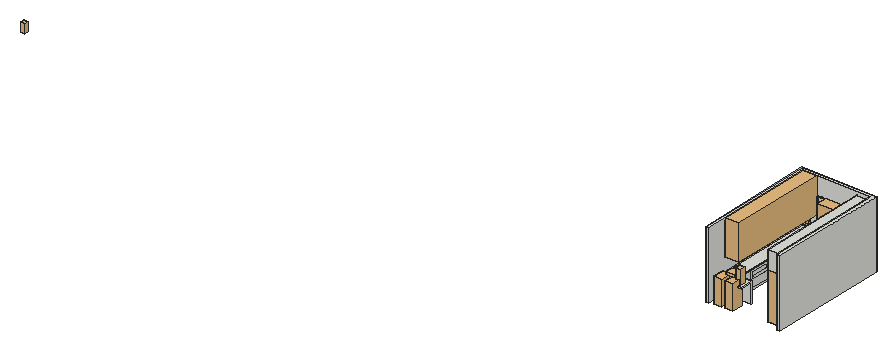
# SketchUp Ruby script. Lengths in inches.
U = 1.inch
M = Sketchup.active_model
def pt(a) = Geom::Point3d.new(a.map { |v| v * U })
def face(e, loops, mat)
  f = e.add_face(loops[0].map { |a| pt(a) })
  loops[1..].each { |l| e.add_face(l.map { |a| pt(a) }).erase! }
  f.material = f.back_material = mat if mat
  f
end
# faces: each face lists its corners as indices into pts; further lists are holes
def faces(e, pts, list, mat = nil) = list.each { |f| face(e, (f[0].is_a?(Array) ? f : [f]).map { |l| l.map { |i| pts[i] } }, mat) }
# xy, xz, yz: faces in a plane at the given z, y or x. An outline is a flat list of corners, or four numbers for a rectangle; further outlines are holes
def ring(l) = l.size == 4 ? [[l[0], l[1]], [l[2], l[1]], [l[2], l[3]], [l[0], l[3]]] : l.each_slice(2).to_a
def flat(e, list, mat, &to3) = list.each { |f| face(e, (f[0].is_a?(Array) ? f : [f]).map { |l| ring(l).map { |u, v| to3.(u, v) } }, mat) }
def xy(e, z, list, mat = nil) = flat(e, list, mat) { |x, y| [x, y, z] }
def xz(e, y, list, mat = nil) = flat(e, list, mat) { |x, z| [x, y, z] }
def yz(e, x, list, mat = nil) = flat(e, list, mat) { |y, z| [x, y, z] }
def lines(e, pts, list) = list.each { |a, b| e.add_line(pt(pts[a]), pt(pts[b])) }
# prism: a flat outline (further loops are holes) pulled along v
def prism(e, loops, v, mat = nil)
  f = face(e, loops, mat); d = Geom::Vector3d.new(v.map { |x| x * U })
  f.pushpull(f.normal.samedirection?(d) ? d.length : -d.length)
end
def box(e, o, s, mat = nil) = prism(e, [[o, [o[0] + s[0], o[1], o[2]], [o[0] + s[0], o[1] + s[1], o[2]], [o[0], o[1] + s[1], o[2]]]], [0, 0, s[2]], mat)
def at(x, y, z, deg = 0) = Geom::Transformation.translation(pt([x, y, z])) * Geom::Transformation.rotation(ORIGIN, Z_AXIS, deg.degrees)
def axes(o, x, y, z) = Geom::Transformation.new([*x, 0, *y, 0, *z, 0, *pt(o).to_a, 1])
def part(name) = M.definitions.add(name)
# library, detail: a bought-in or finely detailed component or shape, given as its bounding box
def library(name, o, s) = part(name).tap { |d| box(d.entities, o, s) }
def detail(e, o, s) = box(e.add_group.entities, o, s)
def put(e, d, t, mat = nil) = e.add_instance(d, t).tap { |i| i.material = mat if mat }
def group(e, t, mat = nil) = e.add_group.tap { |g| g.transformation = t; g.material = mat if mat }.entities
root = M.entities
M.materials.add("4 (5)").color = [147, 109, 57]
M.materials.add("[Translucent Glass Blue]").color = [100, 149, 237]
M.materials["[Translucent Glass Blue]"].alpha = 0.5
c1 = library("Dining chair\#1",[0,0,-0.11],[24.96,20.63,36.01])
c2 = library("Fridge",[0,0,0],[35.75,27.02,77.86])
c3 = part("Sink basin")
detail(c3.entities,[-0.15,-0.15,0],[19.98,14.07,5.91])
c4 = part("Untitled111")
put(c4.entities,c3,at(0.15,0.15,0),"4 (5)")
c5 = library("Blender",[2.53,2.84,0],[8.2,7.51,15.59])
c6 = library("mixer",[2.53,2.84,0],[8.2,7.51,15.59])
c7 = library("Cooker",[0,0,0],[12.41,9.47,7.59])
c8 = library("cooker1",[47.55,-42.3,30.26],[30,24.55,32.96])
c9 = library("5\#2",[-14.24,-10.22,0],[28.4,20.44,1.42])
c10 = library("chimney",[0,0,0],[35.95,27.65,32.08])
c11 = library("decoration wooden - glass bowl",[-0.13,0,1.29],[12.59,10.52,5.85])
c12 = library("Fruit bowl\#1",[0,0,0.08],[19.6875,19.6875,14.09])
c13 = library("Vase_Thin_Flowers",[-6.16,-5.72,0],[9.89,9.25,24.68])
c14 = part("Component\#4")
box(c14.entities,[0,0,0],[35.375,4.125,29.3125])
c15 = library("Knife Set",[-30.69,-30.94,0.125],[10.45,12.99,0.875])
c16 = library("5 STACKED BOWLS",[0,0,0],[6.24,6.24,7.68])
c17 = library("Jar",[0,0,0],[17.5625,21.24,23.15])
c18 = library("Kitchen utensils",[0,-7.04,-2.66],[17.4,17.6,7.97])
c19 = library("Microwave oven",[0,0,0],[23.78,13.12,19.55])
c20 = part("Group19\#1")
p = [[70.8125,1.1875,0],[1.1875,1.1875,0],[1.1875,46.8125,0],[70.8125,46.8125,0]]
lines(c20.entities,p,[[0,1],[1,2],[2,3],[3,0]])
c21 = part("Group18\#1")
prism(c21.entities,[[[72,48,0],[72,0,0],[0,0,0],[0,48,0]],[[1.1875,46.8125,0],[1.1875,1.1875,0],[70.8125,1.1875,0],[70.8125,46.8125,0]]],[0,0,5.875])
put(c21.entities,c20,at(0,0,0))
c22 = library("Group\#8",[30,0,0],[173,24.5,62.5])
xy(root,43.1875,[[54.6875,209,55.6875,214.875],[78.6875,209,78.6875,210.9375,79.1875,210.9375,79.1875,211.9375,78.6875,211.9375,78.6875,214.875,79.6875,214.875,79.6875,209],[31.1875,210.9375,54.6875,211.9375],[55.6875,210.9375,78.6875,211.9375],[78.6875,210.9375,79.1875,211.9375],
  [79.6875,210.9375,102.6875,211.9375],[102.6875,210.9375,103.1875,211.9375]])
xy(root,88.8125,[[54.6875,209,55.6875,214.875],[78.6875,209,79.6875,209,79.6875,214.875,78.6875,214.875,78.6875,211.9375,79.1875,211.9375,79.1875,210.9375,78.6875,210.9375],[31.1875,210.9375,54.6875,211.9375],[55.6875,210.9375,78.6875,211.9375],[78.6875,210.9375,79.1875,211.9375],
  [79.6875,210.9375,102.6875,211.9375],[102.6875,210.9375,103.1875,211.9375]])
xz(root,209,[[54.6875,43.1875,55.6875,88.8125],[78.6875,43.1875,79.6875,88.8125]])
xz(root,210.9375,[[31.1875,43.1875,54.6875,88.8125],[55.6875,43.1875,79.1875,88.8125],[79.6875,43.1875,103.1875,88.8125]])
xz(root,211.9375,[[31.1875,43.1875,54.6875,88.8125],[55.6875,43.1875,79.1875,88.8125],[79.6875,43.1875,103.1875,88.8125]])
xz(root,214.875,[[54.6875,43.1875,55.6875,88.8125],[78.6875,43.1875,79.6875,88.8125]])
yz(root,31.1875,[[210.9375,43.1875,211.9375,88.8125]])
yz(root,54.6875,[[209,43.1875,210.9375,88.8125],[210.9375,43.1875,214.875,88.8125]])
yz(root,55.6875,[[209,43.1875,210.9375,88.8125],[210.9375,43.1875,214.875,88.8125]])
yz(root,78.6875,[[209,43.1875,214.875,88.8125]])
yz(root,79.1875,[[210.9375,43.1875,211.9375,88.8125]])
yz(root,79.6875,[[209,43.1875,210.9375,88.8125],[210.9375,43.1875,214.875,88.8125]])
yz(root,103.1875,[[210.9375,43.1875,211.9375,88.8125]])
p = [[102,106,5],[102,106,82],[101.7,129,82],[101.7,129,5],[30,209,42],[30,209,90],
  [102,209,90],[102,209,42]]
faces(root,p,[[0,1,2,3]],"[Translucent Glass Blue]")
lines(root,p,[[4,5],[6,7],[7,4],[5,6]])
put(root,c1,axes([11.7,2.8125,0.02],[0,0.83304,0],[0.68983,0,0],[0,0,1.2069]))
put(root,c1,axes([31.83,2.8125,0.02],[0,0.83304,0],[0.68983,0,0],[0,0,1.2069]))
put(root,c2,axes([102,57.5,-0.78],[0,-1.28671,0],[0.88823,0,0],[0,0,1.06327]))
put(root,c4,at(100.48,80.02,7.05,-90))
put(root,c5,at(-1225.3125,-0.21,0))
put(root,c6,at(101.31,109.57,51))
put(root,c7,at(102,118.81,67))
put(root,c8,axes([123.29,116.6,0.26],[0,-0.74881,0],[0.50328,0,0],[0,0,0.60256]))
put(root,c9,at(61.42,194.74,34))
put(root,c10,at(46.62,189.4375,57.92))
put(root,c7,at(101.86,108.29,66.72))
put(root,c11,at(107.32,193.84,34))
put(root,c12,axes([20.35,19.08,35.44],[0.8,0,0],[0,0.8,0],[0,0,0.8]))
put(root,c13,axes([45.36,20.66,36],[1,0,0],[0,-1,0],[0,0,1]))
put(root,c14,axes([7.48,208.38,44.77],[0.33217,0,0],[0,0.15,0],[0,0,0.09327]))
put(root,c15,axes([38.45,208.6,70.17],[1,0,0],[0,0,1],[0,-1,0]))
put(root,c16,axes([105.875,113.05,34.99],[1.59,0,0],[0,1.59,0],[0,0,0.9222]))
put(root,c17,axes([110.72,121.59,19],[0.2556,0,0],[0,0.2556,0],[0,0,0.2556]))
put(root,c18,axes([7.16,78,38.95],[0,0,0.77],[0,-0.7182,0],[0.4356,0,0]))
put(root,c19,axes([113.48,58.5,39.05],[0,1,0],[-0.875,0,0],[0,0,1]))
put(root,c17,axes([110.72,113.72,19],[0.2556,0,0],[0,0.2556,0],[0,0,0.2556]))
g1 = group(root,at(6,36,0))
xy(g1,0,[[0,0,0,173,120,173,120,93.5,99,93.5,99,152,21,152,21,0]])
xy(g1,4,[[21,0,24,152],[96,93.5,99,149],[24,149,99,152]])
xy(g1,34,[[0,0,24,0,24,149,96,149,96,93.5,120,93.5,120,173,0,173]])
xz(g1,0,[[0,0,21,0,21,4,24,4,24,34,0,34],[24,33,24.13,33.02,24.25,33.07,24.35,33.15,24.43,33.25,24.48,33.37,24.5,33.5,24.48,33.63,24.43,33.75,24.35,33.85,24.25,33.93,24.13,33.98,24,34]])
xz(g1,93.5,[[99,0,120,0,120,34,96,34,96,4,99,4],[96,33,96,34,95.87,33.98,95.75,33.93,95.65,33.85,95.57,33.75,95.52,33.63,95.5,33.5,95.52,33.37,95.57,33.25,95.65,33.15,95.75,33.07,95.87,33.02]])
xz(g1,149,[[24,4,96,33],[24,33,24,34,24.13,33.98,24.25,33.93,24.35,33.85,24.43,33.75,24.48,33.63,24.5,33.5,24.48,33.37,24.43,33.25,24.35,33.15,24.25,33.07,24.13,33.02],[24,33,24.13,33.02,24.25,33.07,24.35,33.15,24.43,33.25,24.48,33.37,24.5,33.5,24.48,33.63,24.43,33.75,24.35,33.85,24.25,33.93,24.13,33.98,24,34,96,34,95.87,33.98,95.75,33.93,95.65,33.85,95.57,33.75,95.52,33.63,95.5,33.5,95.52,33.37,95.57,33.25,95.65,33.15,95.75,33.07,95.87,33.02,96,33],[96,33,95.87,33.02,95.75,33.07,95.65,33.15,95.57,33.25,95.52,33.37,95.5,33.5,95.52,33.63,95.57,33.75,95.65,33.85,95.75,33.93,95.87,33.98,96,34]])
xz(g1,152,[[21,0,99,4]])
xz(g1,173,[[0,0,120,34]])
yz(g1,0,[[0,0,173,34]])
yz(g1,21,[[0,0,152,4]])
yz(g1,24,[[0,4,149,33],[0,33,149,33,148.87,33.02,148.75,33.07,148.65,33.15,148.57,33.25,148.52,33.37,148.5,33.5,148.52,33.63,148.57,33.75,148.65,33.85,148.75,33.93,148.87,33.98,149,34,0,34],[149,33,149.13,33.02,149.25,33.07,149.35,33.15,149.43,33.25,149.48,33.37,149.5,33.5,149.48,33.63,149.43,33.75,149.35,33.85,149.25,33.93,149.13,33.98,149,34]])
yz(g1,96,[[93.5,4,149,33],[93.5,33,93.5,34,149,34,148.87,33.98,148.75,33.93,148.65,33.85,148.57,33.75,148.52,33.63,148.5,33.5,148.52,33.37,148.57,33.25,148.65,33.15,148.75,33.07,148.87,33.02,149,33]])
yz(g1,99,[[93.5,0,152,4]])
yz(g1,120,[[93.5,0,173,34]])
p = [[24.13,0,33.02],[24,0,33],[24,149,33],[24.13,149,33.02],[24.13,148.87,33.02],[24.25,0,33.07],
  [24.25,149,33.07],[24.25,148.75,33.07],[95.87,93.5,33.02],[95.75,93.5,33.07],[95.75,148.75,33.07],[95.75,149,33.07],
  [95.87,149,33.02],[95.87,148.87,33.02],[96,93.5,33],[96,149,33],[24,148.75,33.07],[24,148.87,33.02],
  [96,148.87,33.02],[96,148.75,33.07],[24.35,0,33.15],[24.35,149,33.15],[24.35,148.65,33.15],[24.43,0,33.25],
  [24.43,149,33.25],[24.43,148.57,33.25],[95.65,93.5,33.15],[95.57,93.5,33.25],[95.57,148.57,33.25],[95.57,149,33.25],
  [95.65,149,33.15],[95.65,148.65,33.15],[24,148.57,33.25],[24,148.65,33.15],[96,148.65,33.15],[96,148.57,33.25],
  [24.48,0,33.37],[24.48,149,33.37],[24.48,148.52,33.37],[95.52,93.5,33.37],[95.52,148.52,33.37],[95.52,149,33.37],
  [24,148.52,33.37],[96,148.52,33.37],[24.5,0,33.5],[24.5,149,33.5],[24.5,148.5,33.5],[95.5,93.5,33.5],
  [95.5,148.5,33.5],[95.5,149,33.5],[24,148.5,33.5],[96,148.5,33.5],[24.48,0,33.63],[24.48,149,33.63],
  [24.48,148.52,33.63],[95.52,93.5,33.63],[95.52,148.52,33.63],[95.52,149,33.63],[24,148.52,33.63],[96,148.52,33.63],
  [24.43,0,33.75],[24.43,149,33.75],[24.43,148.57,33.75],[95.57,93.5,33.75],[95.57,148.57,33.75],[95.57,149,33.75],
  [24,148.57,33.75],[96,148.57,33.75],[24.35,0,33.85],[24.35,149,33.85],[24.35,148.65,33.85],[95.65,93.5,33.85],
  [95.65,148.65,33.85],[95.65,149,33.85],[24,148.65,33.85],[96,148.65,33.85],[24.13,0,33.98],[24.25,0,33.93],
  [24.25,148.75,33.93],[24.25,149,33.93],[24.13,149,33.98],[24.13,148.87,33.98],[95.75,93.5,33.93],[95.75,148.75,33.93],
  [95.75,149,33.93],[95.87,93.5,33.98],[95.87,148.87,33.98],[95.87,149,33.98],[24,148.75,33.93],[96,148.75,33.93],
  [24,148.87,33.98],[96,148.87,33.98],[24,0,34],[24,149,34],[96,93.5,34],[96,149,34]]
faces(g1,p,[[0,1,2,3,4],[5,0,4,3,6,7],[8,9,10,11,12,13],[14,8,13,12,15],[16,17,4,13,18,19,10,7],[17,2,15,18,13,4],[20,5,7,6,21,22],[23,20,22,21,24,25],
  [26,27,28,29,30,31],[9,26,31,30,11,10],[32,33,22,31,34,35,28,25],[33,16,7,10,19,34,31,22],[36,23,25,24,37,38],[27,39,40,41,29,28],[42,32,25,28,35,43,40,38],[44,36,38,37,45,46],
  [39,47,48,49,41,40],[50,42,38,40,43,51,48,46],[52,44,46,45,53,54],[47,55,56,57,49,48],[58,50,46,48,51,59,56,54],[60,52,54,53,61,62],[55,63,64,65,57,56],[66,58,54,56,59,67,64,62],
  [68,60,62,61,69,70],[63,71,72,73,65,64],[74,66,62,64,67,75,72,70],[76,77,78,79,80,81],[77,68,70,69,79,78],[71,82,83,84,73,72],[82,85,86,87,84,83],[88,74,70,72,75,89,83,78],
  [90,88,78,83,89,91,86,81],[92,76,81,80,93],[85,94,95,87,86],[93,90,81,86,91,95]])
g2 = group(root,at(30,185.1,4))
xy(g2,0,[[0.5,-0.3,20.5,0],[21.5,-0.3,51.5,0],[52.5,-0.3,71,0],[0,-0.1,0.5,0],[20.5,-0.1,21.5,0],
  [51.5,-0.1,52.5,0],[71,-0.1,72,0]])
xy(g2,11.5,[[21.5,-0.3,51.5,-0.1]])
xy(g2,12.5,[[21.5,-0.3,51.5,-0.1]])
xy(g2,20.5,[[21.5,-0.3,51.5,-0.1],[52.5,-0.3,71,-0.1]])
xy(g2,21.5,[[21.5,-0.3,51.5,-0.1],[52.5,-0.3,71,-0.1]])
xy(g2,27.5,[[0.5,-0.3,11.5,-0.1],[11.5,-0.3,20.5,-0.1],[21.5,-0.3,51.5,-0.1],[52.5,-0.3,71,-0.1]])
xy(g2,29,[[0,-0.1,0.5,0],[0.5,-0.1,11.5,0],[11.5,-0.1,20.5,0],[20.5,-0.1,21.5,0],[21.5,-0.1,51.5,0],
  [51.5,-0.1,52.5,0],[52.5,-0.1,71,0],[71,-0.1,72,0]])
xz(g2,-0.3,[[0.5,0,20.5,27.5],[21.5,0,51.5,11.5],[52.5,0,71,20.5],[21.5,12.5,51.5,20.5],[21.5,21.5,51.5,27.5],
  [52.5,21.5,71,27.5]])
xz(g2,-0.1,[[[0,0,0.5,0,0.5,27.5,20.5,27.5,20.5,0,21.5,0,21.5,11.5,51.5,11.5,51.5,0,52.5,0,52.5,20.5,71,20.5,71,0,72,0,72,29,0,29],[21.5,12.5,51.5,20.5],[21.5,21.5,51.5,27.5],[52.5,21.5,71,27.5]]])
xz(g2,0,[[0,0,0.5,29]])
yz(g2,0,[[-0.1,0,0,29]])
yz(g2,0.5,[[-0.3,0,-0.1,27.5]])
yz(g2,20.5,[[-0.3,0,-0.1,27.5]])
yz(g2,21.5,[[-0.3,0,-0.1,11.5],[-0.3,12.5,-0.1,20.5],[-0.3,21.5,-0.1,27.5]])
yz(g2,51.5,[[-0.3,0,-0.1,11.5],[-0.3,12.5,-0.1,20.5],[-0.3,21.5,-0.1,27.5]])
yz(g2,52.5,[[-0.3,0,-0.1,20.5],[-0.3,21.5,-0.1,27.5]])
yz(g2,71,[[-0.3,0,-0.1,20.5],[-0.3,21.5,-0.1,27.5]])
yz(g2,72,[[-0.1,0,0,28.5],[-0.1,28.5,0,29]])
p = [[0.5,0,28.5],[0.5,-0.1,28.5],[0.5,0,27.5],[0.5,-0.1,27.5]]
lines(g2,p,[[0,1],[2,3]])
g3 = group(root,at(30,36,0))
xy(g3,0,[[0,24.5,0.1,66.5]])
xy(g3,4,[[0,0,0,24.5,0.1,24.5,0.1,23.5,0.3,23.5,0.3,0],[0.1,24.5,0.3,66.5],[0,66.5,0,87.5,0.1,87.5,0.1,87,0.3,87,0.3,67.5,0.1,67.5,0.1,66.5],[0,87.5,0,110,0.1,110,0.1,109.5,0.3,109.5,0.3,88.01,0.1,88.01,0.1,87.5],[0,110,0,130.5,0.1,130.5,0.1,130,0.3,130,0.3,110.5,0.1,110.5,0.1,110],
  [0,130.5,0,149,0.3,149,0.3,131,0.1,131,0.1,130.5]])
xy(g3,17,[[0.1,0,0.3,23.5],[0.1,24.5,0.3,66.5],[0.1,67.5,0.3,87],[0.1,88.01,0.3,109.5],[0.1,110.5,0.3,130],
  [0.1,131,0.3,149]])
xy(g3,18,[[0.1,0,0.3,23.5],[0.1,24.5,0.3,66.5],[0.1,110.5,0.3,130],[0.1,131,0.3,149]])
xy(g3,18.5,[[0.1,67.5,0.3,87],[0.1,88.01,0.3,109.5]])
xy(g3,22.3125,[[0.1,29.125,0.3,62.12]])
xy(g3,29.12,[[0.1,29.125,0.3,62.12]])
xy(g3,32,[[0.1,0,0.3,23.5],[0.1,67.5,0.3,87],[0.1,88,0.3,109.5],[0.1,110.5,0.3,130],[0.1,131,0.3,149]])
xy(g3,33,[[0,0,0.1,24.5],[0,24.5,0.3,66.5],[0,66.5,0.1,87.5],[0,87.5,0.1,110],[0,110,0.1,130.5],
  [0,130.5,0.1,149]])
xz(g3,0,[[0,4,0.3,4,0.3,17,0.1,17,0.1,17.5,0,17.5],[0,17.5,0.1,17.5,0.1,18,0.3,18,0.3,32,0,32],[0,32,0.1,33]])
xz(g3,23.5,[[0.1,4,0.3,17],[0.1,18,0.3,32]])
xz(g3,24.5,[[0,0,0.1,4],[0.1,4,0.3,17],[0.1,18,0.3,32],[0.1,32,0.3,33]])
xz(g3,29.125,[[0.1,22.3125,0.3,29.12]])
xz(g3,62.12,[[0.1,22.3125,0.3,29.12]])
xz(g3,66.5,[[0,0,0.1,4],[0.1,4,0.3,17],[0.1,18,0.3,18.5],[0.1,18.5,0.3,32],[0.1,32,0.3,33]])
xz(g3,67.5,[[0.1,4,0.3,17],[0.1,18.5,0.3,32]])
xz(g3,87,[[0.1,4,0.3,17],[0.1,18.5,0.3,32]])
xz(g3,88.01,[[0.1,4,0.3,17]])
xz(g3,109.5,[[0.1,4,0.3,17],[0.1,18.5,0.3,32]])
xz(g3,110.5,[[0.1,4,0.3,17],[0.1,18,0.3,32]])
xz(g3,130,[[0.1,4,0.3,17],[0.1,18,0.3,32]])
xz(g3,131,[[0.1,4,0.3,17],[0.1,18,0.3,32]])
xz(g3,149,[[0,4,0,32,0.3,32,0.3,18,0.1,18,0.1,17,0.3,17,0.3,4],[0,32,0.1,33]])
yz(g3,0,[[0,4,24.5,17.5]])
yz(g3,0.1,[[24.5,0,66.5,4],[[23.5,4,24.5,4,24.5,17,66.5,17,66.5,4,67.5,4,67.5,17,87,17,87,4,88.01,4,88.01,17,109.5,17,109.5,4,110.5,4,110.5,17,130,17,130,4,131,4,131,17,149,17,149,18,131,18,131,32,149,32,149,33,66.5,33,66.5,18,24.5,18,24.5,33,0,33,0,32,23.5,32,23.5,18,0,18,0,17,23.5,17],[88.01,18.5,88,32,109.5,32,109.5,18.5],[110.5,18,130,32],[67.5,18.5,87,32]],[29.125,22.3125,62.12,29.12]])
yz(g3,0.3,[[0,4,23.5,17],[24.5,4,66.5,17],[67.5,4,87,17],[88.01,4,109.5,17],[110.5,4,130,17],
  [131,4,149,17],[0,18,23.5,32],[[24.5,18,66.5,33],[29.125,22.3125,62.12,29.12]],[110.5,18,130,32],[131,18,149,32],
  [67.5,18.5,87,32],[88.01,18.5,109.5,18.5,109.5,32,88,32]])
p = [[0.1,88,32],[0.1,88.01,18.5],[0.3,88.01,18.5],[0.3,88,32]]
faces(g3,p,[[0,1,2,3]])
g4 = group(root,at(102.1,185,4))
xy(g4,0,[[-0.4,-55.5,0,-25.5],[-0.1,-25.5,-0.1,-24.5,-0.4,-24.5,-0.4,0,0,0,0,-25.5]])
xy(g4,13.5,[[-0.4,-55.5,-0.1,-25.5],[-0.1,-55.5,0,-25.5]])
xy(g4,14.5,[[-0.4,-55.5,-0.1,-25.5]])
xy(g4,28,[[-0.4,-55.5,-0.1,-25.5],[-0.1,-55.5,0,-25.5],[-0.4,-24.5,-0.1,0]])
xy(g4,29,[[-0.1,-55.5,0,-25.5],[-0.1,-25.5,0,0]])
xz(g4,-55.5,[[-0.4,0,0,13.5],[-0.1,13.5,0,14.5],[-0.4,14.5,0,28],[-0.1,28,0,29]])
xz(g4,-25.5,[[-0.4,0,-0.1,13.5],[-0.1,0,0,13.5],[-0.4,14.5,-0.1,28],[-0.1,14.5,0,28]])
xz(g4,-24.5,[[-0.4,0,-0.1,28]])
xz(g4,0,[[-0.4,0,0,28],[-0.1,28,0,29]])
yz(g4,-0.4,[[-55.5,0,-25.5,13.5],[-24.5,0,0,28],[-55.5,14.5,-25.5,28]])
yz(g4,-0.1,[[-25.5,0,-25.5,13.5,-55.5,13.5,-55.5,14.5,-25.5,14.5,-25.5,28,-55.5,28,-55.5,29,0,29,0,28,-24.5,28,-24.5,0]])
yz(g4,0,[[-55.5,0,-25.5,13.5],[-25.5,0,0,28],[-55.5,14.5,-25.5,28],[-55.5,28,-25.5,29],[-25.5,28,0,29]])
g5 = group(root,at(27,60.5,0))
xz(g5,0,[[0,0,3,4]])
xz(g5,42,[[0,0,3,4]])
g6 = group(root,at(126,209,0))
xy(g6,0,[[-21,-151.5,0,-79.5]])
xy(g6,4,[[-24,-151.5,-21,-127.5],[-24,-127.5,-21,-103.5],[-21,-127.5,0,-103.5],[-24,-103.5,-21,-79.5]])
xy(g6,5,[[-24,-150.5,-6,-128],[-24,-103,-6,-80]])
xy(g6,17.5,[[-24,-150.5,-6,-128]])
xy(g6,18,[[-24,-103,-6,-80]])
xy(g6,18.5,[[-24,-150.5,-6,-128]])
xy(g6,19,[[-24,-103,-6,-80]])
xy(g6,34,[[-24,-103,-6,-80]])
xy(g6,35,[[-24,-103,-6,-80]])
xy(g6,38.05,[[-24,-150.5,-6,-128]])
xy(g6,39.05,[[-24,-150.5,-6,-128]])
xy(g6,50,[[-24,-103,-6,-80]])
xy(g6,51,[[-24,-103,-6,-80]])
xy(g6,57.59,[[-24,-150.5,-6,-128]])
xy(g6,58,[[-12.3,-79.5,-12.3,-60.5,-12,-60.5,-12,-59.5,-12.3,-59.5,-12.3,-40.5,-12,-40.5,-12,-39.5,-12.3,-39.5,-12.3,-20.5,-12,-20.5,-12,-19.5,-12.3,-19.5,-12.3,0,0,0,0,-79.5]])
xy(g6,66,[[-24,-103,-6,-80]])
xy(g6,67,[[-24,-103,-6,-80]])
xy(g6,82,[[-24.3,-197.5,-24.3,-175,-24,-175,-24,-174,-24.3,-174,-24.3,-151.5,0,-151.5,0,-197.5],[-24.3,-150.5,-24,-128],[-24.3,-127,-24,-104],[-24.3,-103,-6,-80],[-24,-79.5,-24,-79,-24.3,-79,-24.3,-60.5,-24,-60.5,-24,-59.5,-24.3,-59.5,-24.3,-40.5,-24,-40.5,-24,-39.5,-24.3,-39.5,-24.3,-20.5,-24,-20.5,-24,-19.5,-24.3,-19.5,-24.3,0,-12.3,0,-12.3,-19.5,-12,-19.5,-12,-20.5,-12.3,-20.5,-12.3,-39.5,-12,-39.5,-12,-40.5,-12.3,-40.5,-12.3,-59.5,-12,-59.5,-12,-60.5,-12.3,-60.5,-12.3,-79.5]])
xy(g6,114,[[-24.3,-197.5,0,-197.5,0,0,-24.3,0,-24.3,-19.5,-24,-19.5,-24,-20.5,-24.3,-20.5,-24.3,-39.5,-24,-39.5,-24,-40.5,-24.3,-40.5,-24.3,-59.5,-24,-59.5,-24,-60.5,-24.3,-60.5,-24.3,-79,-24,-79,-24,-80,-24.3,-80,-24.3,-103,-24,-103,-24,-104,-24.3,-104,-24.3,-127,-24,-127,-24,-128,-24.3,-128,-24.3,-150.5,-24,-150.5,-24,-151.5,-24.3,-151.5,-24.3,-174,-24,-174,-24,-175,-24.3,-175]])
xz(g6,-197.5,[[-24.3,82,0,114]])
xz(g6,-175,[[-24.3,82,-24,114]])
xz(g6,-174,[[-24.3,82,-24,114]])
xz(g6,-151.5,[[-21,0,0,0,0,82,-24,82,-24,4,-21,4],[-24.3,82,-24,114]])
xz(g6,-150.5,[[-24,5,-6,17.5],[-24,18.5,-6,38.05],[-24,39.05,-6,57.59],[-24.3,82,-24,114]])
xz(g6,-128,[[-24,5,-6,17.5],[-24,18.5,-6,38.05],[-24,39.05,-6,57.59],[-24.3,82,-24,114]])
xz(g6,-127,[[-24.3,82,-24,114]])
xz(g6,-104,[[-24.3,82,-24,114]])
xz(g6,-103,[[-24,5,-6,18],[-24,19,-6,34],[-24,35,-6,50],[-24,51,-6,66],[-24,67,-6,82],
  [-24.3,82,-24,114]])
xz(g6,-80,[[-24,5,-6,18],[-24,19,-6,34],[-24,35,-6,50],[-24,51,-6,66],[-24,67,-6,82],
  [-24.3,82,-24,114]])
xz(g6,-79.5,[[-21,0,-21,4,-24,4,-24,82,-12.3,82,-12.3,58,0,58,0,0]])
xz(g6,-79,[[-24.3,82,-24,114]])
xz(g6,-60.5,[[-12.3,58,-12,82],[-24.3,82,-24,114]])
xz(g6,-59.5,[[-12.3,58,-12,82],[-24.3,82,-24,114]])
xz(g6,-40.5,[[-12.3,58,-12,82],[-24.3,82,-24,114]])
xz(g6,-39.5,[[-12.3,58,-12,82],[-24.3,82,-24,114]])
xz(g6,-20.5,[[-12.3,58,-12,82],[-24.3,82,-24,114]])
xz(g6,-19.5,[[-12.3,58,-12,82],[-24.3,82,-24,114]])
xz(g6,0,[[-12.3,58,-12.3,82,-24.3,82,-24.3,114,0,114,0,58]])
yz(g6,-24.3,[[-197.5,82,-175,114],[-174,82,-151.5,114],[-150.5,82,-128,114],[-127,82,-104,114],[-103,82,-80,114],
  [-79,82,-60.5,114],[-59.5,82,-40.5,114],[-39.5,82,-20.5,114],[-19.5,82,0,114]])
yz(g6,-24,[[-151.5,4,-150.5,17.5],[-150.5,4,-128,5],[-128,4,-127.5,5],[-127.5,4,-127,5],[-127,4,-104,5],
  [-104,4,-103.5,5],[-103.5,4,-103,5],[-103,4,-80,5],[-80,4,-79.5,18],[-128,5,-127.5,17.5],
  [-127.5,5,-127,82],[-127,5,-104,82],[-104,5,-103.5,82],[-103.5,5,-103,82],[-151.5,17.5,-150.5,18.5],
  [-150.5,17.5,-128,18.5],[-128,17.5,-127.5,18.5],[-103,18,-80,19],[-80,18,-79.5,19],[-151.5,18.5,-150.5,38.05],
  [-128,18.5,-127.5,38.05],[-80,19,-79.5,34],[-103,34,-80,35],[-80,34,-79.5,35],[-80,35,-79.5,50],
  [-151.5,38.05,-150.5,39.05],[-150.5,38.05,-128,39.05],[-128,38.05,-127.5,57.59],[-151.5,39.05,-150.5,57.59],[-103,50,-80,51],
  [-80,50,-79.5,51],[-80,51,-79.5,66],[-151.5,57.59,-150.5,58.59],[-150.5,57.59,-128,58.59],[-128,57.59,-127.5,82],
  [-151.5,58.59,-150.5,82],[-150.5,58.59,-128,82],[-103,66,-80,67],[-80,66,-79.5,67],[-80,67,-79.5,82],
  [-175,82,-174.5,114],[-174.5,82,-174,114],[-151.5,82,-151,114],[-151,82,-150.5,114],[-128,82,-127.5,114],
  [-127.5,82,-127,114],[-104,82,-103.5,114],[-103.5,82,-103,114],[-80,82,-79.5,114],[-79.5,82,-79,114],
  [-60.5,82,-60,114],[-60,82,-59.5,114],[-40.5,82,-40,114],[-40,82,-39.5,114],[-20.5,82,-19.5,114]])
yz(g6,-21,[[-151.5,0,-79.5,4]])
yz(g6,-12.3,[[-79.5,58,-60.5,82],[-59.5,58,-40.5,82],[-39.5,58,-20.5,82],[-19.5,58,0,82]])
yz(g6,-12,[[-60.5,58,-59.5,82],[-40.5,58,-39.5,82],[-20.5,58,-19.5,82]])
yz(g6,-6,[[-150.5,5,-128,17.5],[-103,5,-80,18],[-150.5,18.5,-128,38.05],[-103,19,-80,34],[-103,35,-80,50],
  [-150.5,39.05,-128,57.59],[-103,51,-80,66],[-103,67,-80,82]])
yz(g6,0,[[-151.5,0,-79.5,4],[-151.5,4,-151.5,82,-197.5,82,-197.5,114,0,114,0,58,-79.5,58,-79.5,4],[-197.5,114,0,120]])
g7 = group(root,at(0,12,0))
xy(g7,0,[[0,-12,0,203,132,203,132,-12,126,-12,126,197,6,197,6,-12]])
xy(g7,42,[[30,197,102,203]])
xy(g7,90,[[30,197,102,203]])
xy(g7,120,[[0,-12,6,-12,6,197,126,197,126,-12,132,-12,132,203,0,203]])
xz(g7,-12,[[0,0,6,120],[126,0,132,120]])
xz(g7,197,[[[6,0,126,120],[30,42,102,90]]])
xz(g7,203,[[[0,0,132,120],[30,42,102,90]]])
yz(g7,0,[[-12,0,203,120]])
yz(g7,6,[[-12,0,197,120]])
yz(g7,30,[[197,42,203,90]])
yz(g7,102,[[197,42,203,90]])
yz(g7,126,[[-12,0,197,120]])
yz(g7,132,[[-12,0,203,120]])
put(root,c21,axes([30,214.875,42],[1,0,0],[0,0,1],[0,-1,0]))
put(root,c22,at(30.5,6,58,90))
g8 = group(root,at(6,12,0))
prism(g8,[[[48,0,34],[48,22,34],[48,22,0],[48,24,0],[48,24,36],[48,0,36]]],[-48,0,0])
